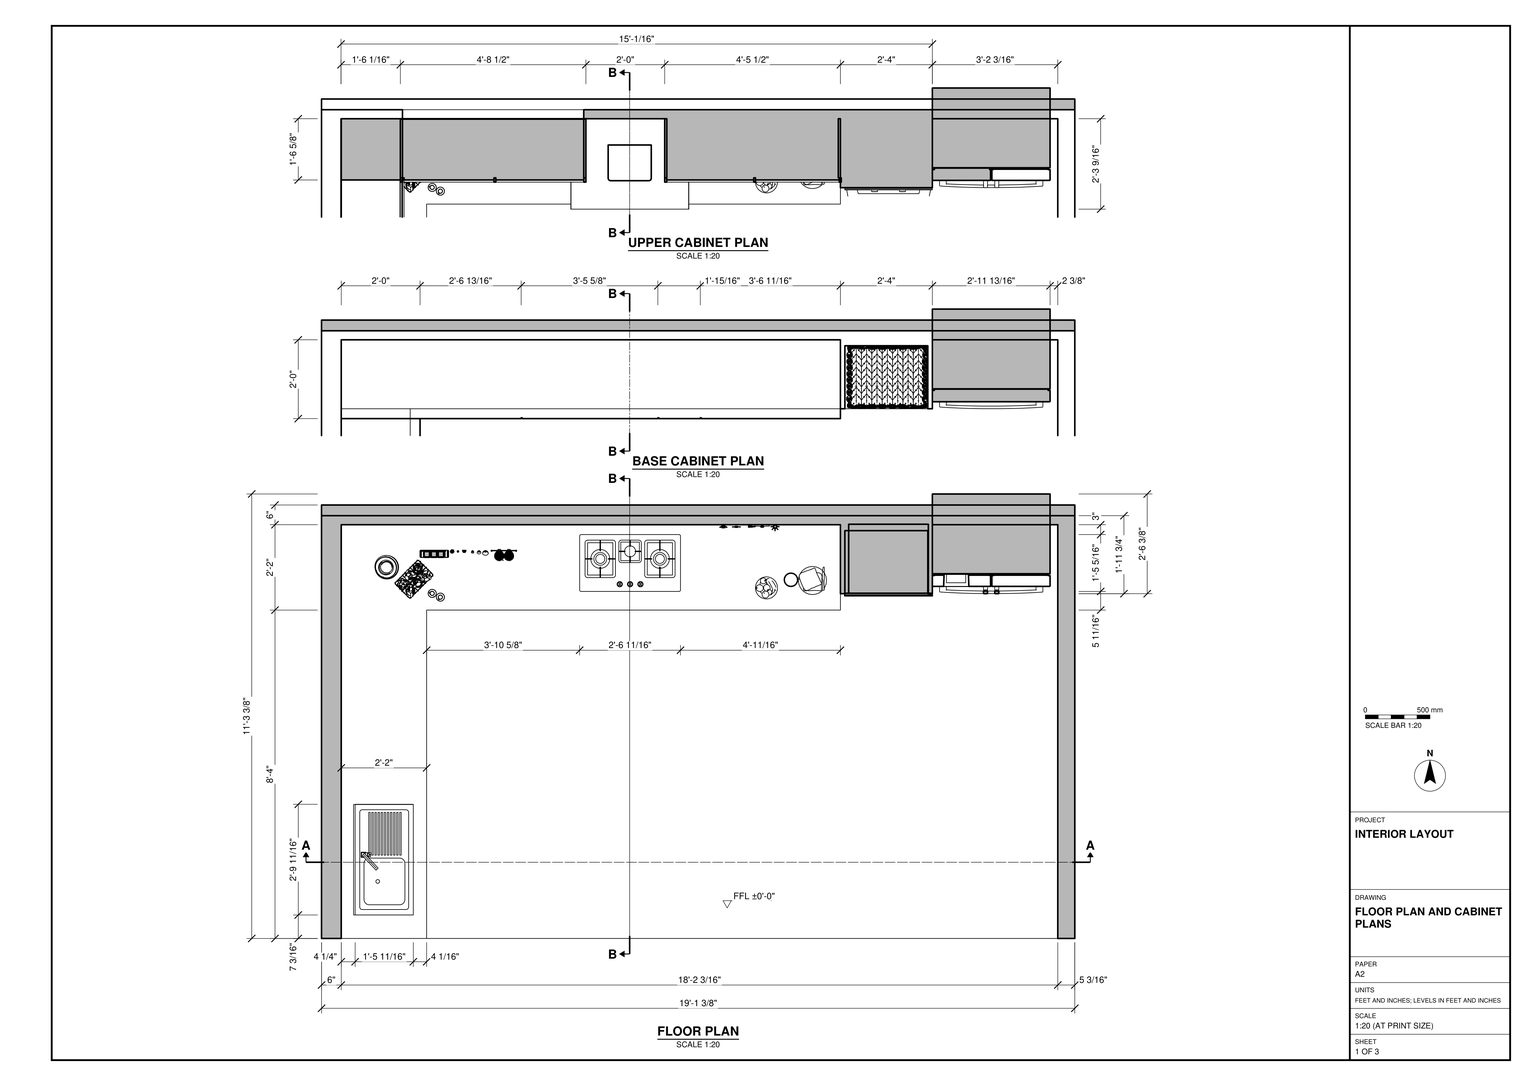
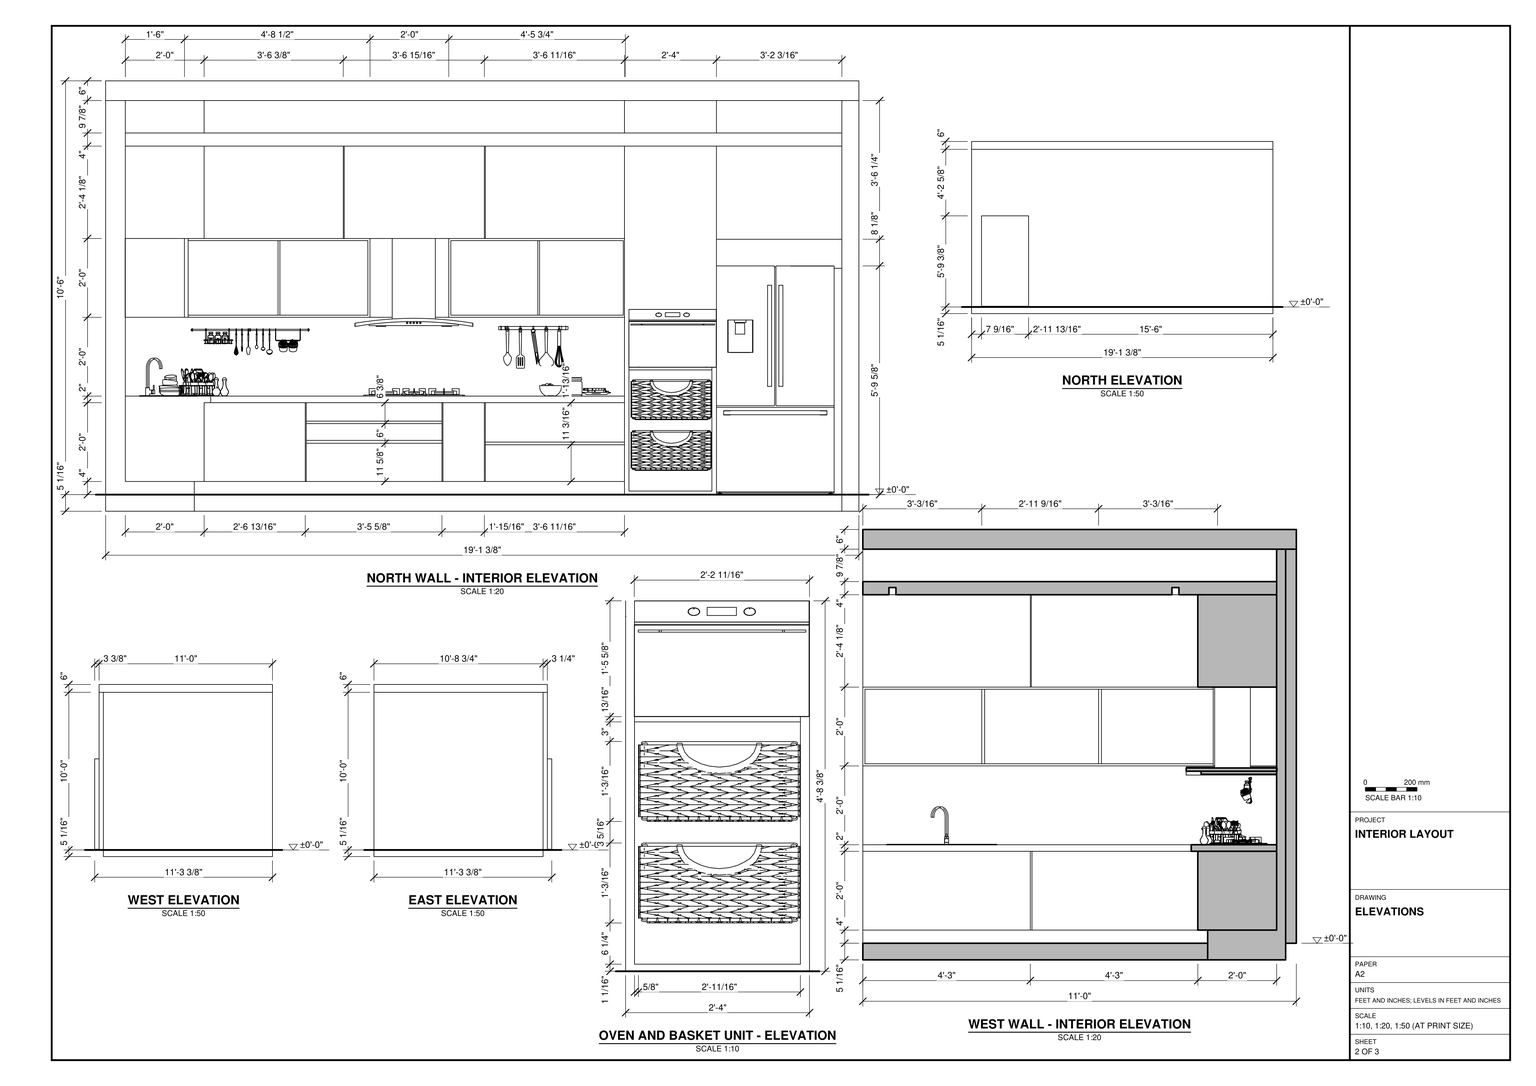
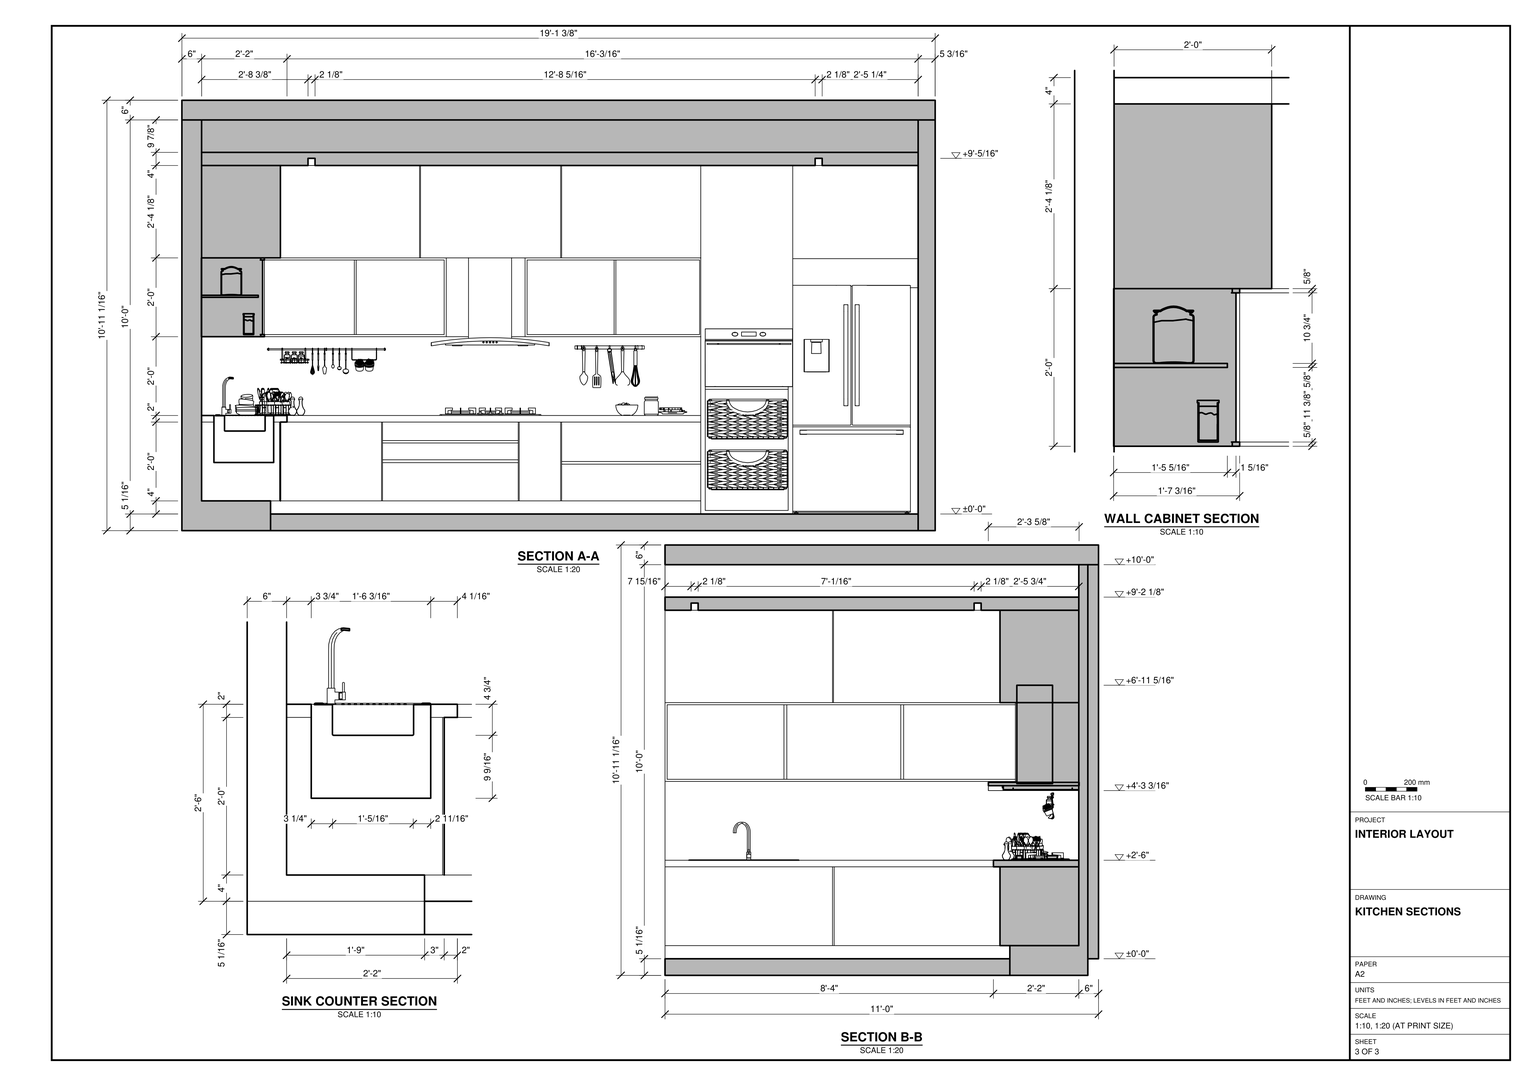
Build the kitchen interior in SketchUp using task_files/diagram_01.pdf. Work in feet and inches. The complete model measures 37'-4 9/16" along X, 24'-8 9/16" along Y and 10'-11 1/16" along Z. Set the finished floor of the single storey at ±0'-0". Use the local plan dimensions for the kitchen itself: the enclosure measures 19'-1 3/8" across the north wall. Model the floor slab, overhead slab, ceiling detail and three enclosing walls at their drawn thicknesses, leaving the south side open as shown.

Fit a continuous L-shaped worktop along the north and west walls. Use the cabinet plans for the depths and the interior elevations for the cupboard fronts, drawer divisions and recessed plinth. Place the sink, draining board and tap near the open end of the west return. Align the cooktop on the north run with the hood in the gap between the wall cabinets. Follow the wall cabinet section for the change in depth between tiers. At the east end of the north run, fit the oven unit with baskets beneath it and place the refrigerator in the adjoining end bay.

Decor and loose items, including appliances, hanging utensils and countertop accessories, may be represented by any suitable library components. Keep shell elements and individual furniture or joinery pieces in separate groups or components, and use components for repeated parts. Save one SketchUp model as output_files/l_shaped_fitted_kitchen_and_its_room_enclosure.skp.

# SketchUp Ruby script. Lengths in inches.
U = 1.inch
M = Sketchup.active_model
def pt(a) = Geom::Point3d.new(a.map { |v| v * U })
def face(e, loops, mat)
  f = e.add_face(loops[0].map { |a| pt(a) })
  loops[1..].each { |l| e.add_face(l.map { |a| pt(a) }).erase! }
  f.material = f.back_material = mat if mat
  f
end
# faces: each face lists its corners as indices into pts; further lists are holes
def faces(e, pts, list, mat = nil) = list.each { |f| face(e, (f[0].is_a?(Array) ? f : [f]).map { |l| l.map { |i| pts[i] } }, mat) }
# xy, xz, yz: faces in a plane at the given z, y or x. An outline is a flat list of corners, or four numbers for a rectangle; further outlines are holes
def ring(l) = l.size == 4 ? [[l[0], l[1]], [l[2], l[1]], [l[2], l[3]], [l[0], l[3]]] : l.each_slice(2).to_a
def flat(e, list, mat, &to3) = list.each { |f| face(e, (f[0].is_a?(Array) ? f : [f]).map { |l| ring(l).map { |u, v| to3.(u, v) } }, mat) }
def xy(e, z, list, mat = nil) = flat(e, list, mat) { |x, y| [x, y, z] }
def xz(e, y, list, mat = nil) = flat(e, list, mat) { |x, z| [x, y, z] }
def yz(e, x, list, mat = nil) = flat(e, list, mat) { |y, z| [x, y, z] }
def lines(e, pts, list) = list.each { |a, b| e.add_line(pt(pts[a]), pt(pts[b])) }
# prism: a flat outline (further loops are holes) pulled along v
def prism(e, loops, v, mat = nil)
  f = face(e, loops, mat); d = Geom::Vector3d.new(v.map { |x| x * U })
  f.pushpull(f.normal.samedirection?(d) ? d.length : -d.length)
end
def box(e, o, s, mat = nil) = prism(e, [[o, [o[0] + s[0], o[1], o[2]], [o[0] + s[0], o[1] + s[1], o[2]], [o[0], o[1] + s[1], o[2]]]], [0, 0, s[2]], mat)
def at(x, y, z, deg = 0) = Geom::Transformation.translation(pt([x, y, z])) * Geom::Transformation.rotation(ORIGIN, Z_AXIS, deg.degrees)
def axes(o, x, y, z) = Geom::Transformation.new([*x, 0, *y, 0, *z, 0, *pt(o).to_a, 1])
def part(name) = M.definitions.add(name)
# library, detail: a bought-in or finely detailed component or shape, given as its bounding box
def library(name, o, s) = part(name).tap { |d| box(d.entities, o, s) }
def detail(e, o, s) = box(e.add_group.entities, o, s)
def put(e, d, t, mat = nil) = e.add_instance(d, t).tap { |i| i.material = mat if mat }
def group(e, t, mat = nil) = e.add_group.tap { |g| g.transformation = t; g.material = mat if mat }.entities
root = M.entities
M.materials.add("[0085_Turquoise]").color = [48, 112, 112]
M.materials.add("[0132_LightGray]").color = [169, 169, 169]
M.materials.add("[0135_DarkGray]").color = [51, 51, 51]
M.materials["[0135_DarkGray]"].alpha = 0.48
M.materials.add("[0136_Charcoal]").color = [33, 33, 33]
M.materials.add("[0136_Charcoal]1").color = [35, 35, 35]
M.materials.add("[0137_Black]").color = [0, 0, 0]
M.materials.add("[Tile Limestone Large]").color = [249, 242, 237]
M.materials.add("[Wax 02]").color = [189, 234, 186]
M.materials.add("cnwhc.com_草图联盟_1kmauOsh").color = [54, 52, 52]
M.materials.add("cnwhc.com_草图联盟_C8Y5Xp2O").color = [156, 156, 156]
M.materials["cnwhc.com_草图联盟_C8Y5Xp2O"].alpha = 0.15
M.materials.add("cnwhc.com_草图联盟_IHFcDxe1").color = [138, 151, 59]
M.materials.add("cnwhc.com_草图联盟_KNEfX85g").color = [162, 126, 87]
M.materials.add("cnwhc.com_草图联盟_QJow1Ky4").color = [144, 133, 65]
M.materials.add("cnwhc.com_草图联盟_z6N5x4Hv").color = [223, 205, 124]
c1 = library("Cup rack\#1",[0,0,0],[12.28,12.62,7.74])
c2 = library("Food+jars (1)",[-3.15,-4.1,0],[15.4,16.05,11.47])
c3 = library("Group\#13",[-397.46,82.38,-0.11],[62.88,62.86,260])
c4 = library("Group\#14",[-282.65,82.375,-0.11],[62.85,62.875,260.02])
c5 = library("Group\#15",[222.96,189.98,-0.44],[259.48,39.25,337.49])
c6 = library("Group\#30",[41.52,-158.49,40.25],[95.93,90.14,172.87])
c7 = library("Group\#21",[-504.125,120.57,-0.1],[108.2,108.21,338.13])
c8 = library("Group\#22",[-376.9,120.94,-0.1],[107.79,107.8,326.37])
c9 = library("Group\#23",[-254.81,120.48,-0.6],[108.21,108.21,334.5])
c10 = library("Group\#24",[-133.01,121.19,-0.1],[106.95,106.95,324.89])
c11 = library("Group\#25",[0.46,121.12,-0.1],[106.94,106.94,338.14])
c12 = library("Group\#26",[151.35,137.54,-0.1],[70.51,70.14,256.45])
c13 = library("Group\#27",[-266.02,-201.27,40.23],[225.02,228.69,89.38])
c14 = library("Group\#28",[-78.56,-74.98,40.25],[131.28,107.59,245.3125])
c15 = library("Group\#31",[-60.55,-181.2,40.41],[105.85,106.35,65.49])
c16 = library("Group\#34",[253.59,42.68,151.97],[53.13,53.13,100.94])
c17 = library("Group\#35",[281.12,-5,151.97],[53.13,53.13,100.92])
c18 = library("Group\#36",[308.75,-52.85,151.97],[53.125,53.13,100.94])
c19 = library("Group\#37",[336.19,-100.38,151.98],[53.13,53.13,100.93])
c20 = library("Group\#38",[363.79,-148.1875,151.98],[53.13,53.13,100.93])
c21 = library("Group\#39",[253.59,42.68,30.7],[53.13,53.13,100.93])
c22 = library("Group\#40",[281.12,-5,30.7],[53.13,53.13,100.91])
c23 = library("Group\#41",[308.75,-52.85,30.7],[53.125,53.13,100.94])
c24 = library("Group\#42",[336.19,-100.38,30.7],[53.13,53.13,100.91])
c25 = library("Group\#43",[363.79,-148.1875,30.7],[53.13,53.13,100.93])
c26 = library("Group\#44",[212.54,-198.04,-0.24],[263.36,352.65,298.47])
c27 = library("Group\#29",[55.69,-19.19,40.37],[80.08,80.05,323.81])
c28 = part("KITCHEN+ITEMS+(1)")
put(c28.entities,c3,at(0,0,0))
put(c28.entities,c4,at(0,0,0))
put(c28.entities,c5,at(0,0,0))
put(c28.entities,c6,at(0,0,-41.3))
put(c28.entities,c7,at(0,0,0))
put(c28.entities,c8,at(0,0,0))
put(c28.entities,c9,at(0,0,0))
put(c28.entities,c10,at(0,0,0))
put(c28.entities,c11,at(0,0,0))
put(c28.entities,c12,at(0,0,0))
put(c28.entities,c13,at(0,0,-41.3))
put(c28.entities,c14,at(0,0,-41.3))
put(c28.entities,c15,at(0,0,-41.3))
put(c28.entities,c16,at(0,0,0))
put(c28.entities,c17,at(0,0,0))
put(c28.entities,c18,at(0,0,0))
put(c28.entities,c19,at(0,0,0))
put(c28.entities,c20,at(0,0,0))
put(c28.entities,c21,at(0,0,0))
put(c28.entities,c22,at(0,0,0))
put(c28.entities,c23,at(0,0,0))
put(c28.entities,c24,at(0,0,0))
put(c28.entities,c25,at(0,0,0))
put(c28.entities,c26,at(0,0,0))
put(c28.entities,c27,at(0,0,-41.3))
c29 = library("Tableware assortment",[-1.93,-1.45,-0.01],[13.28,36.8,12.14])
c30 = library("Food+jars (2)",[-11.5,-3.52,0],[30.82,7.02,10])
c31 = library("Food+jars",[176.18,154.2,55.15],[6.14,23.65,7.76])
c32 = library("Stack of bowls \#1",[0,0,0],[8.98,8.99,10.96])
c33 = library("Oven",[-9.26,-22.59,0.07],[23.42,23.91,23.21])
c34 = library("Library component",[0.34,0,0],[62.86,27.86,1.18])
c35 = library("Woven storage basket",[0,0,0],[10.23,12.78,4.26])
c36 = library("B36CD50SNS_tradeCAD",[0,0,0],[35.84,30.35,69.65])
c37 = library("Bread1",[0,0,0],[12.98,8.57,5.62])
c38 = library("vm_v2_031",[-4.73,-4.73,0],[9.46,9.46,3.85])
c39 = library("Component_12",[0,0,0],[17.72,31.5,20.63])
c40 = library("Kitchen Utensil.",[-24.86,-2.29,-26.5],[81.83,11.85,18.87])
c41 = library("skpC936",[0,-1.9,0],[21.12,3.04,12.85])
c42 = library("PV977NSS_GEProfile",[-17.9375,-27.5625,-0.25],[35.95,27.64,32.08])
c43 = library("Group\#88",[-453.95,-270.9,-0.08],[243.89,243.63,216.82])
c44 = library("Group\#68",[118.34,-437.05,68.8],[33.09,42.97,27.32])
c45 = library("Group\#69",[91.875,-459.8125,1.36],[84.84,84.82,167.94])
c46 = library("Group\#70",[93.63,-458.06,3.28],[81.33,81.31,90.04])
c47 = library("Group\#71",[114.46,-437.1875,150.05],[39.68,39.57,39.67])
c48 = library("Group\#72",[177.52,-496.26,3.28],[81.21,81.23,127.94])
c49 = library("Group\#73",[175.77,-498.01,1.36],[84.71,84.74,167.94])
c50 = library("Group\#74",[198.24,-475.92,149.53],[39.78,40.55,40.71])
c51 = library("Group\#75",[-248.47,-468.28,0.39],[392.05,393.05,278.56])
c52 = library("Group\#76",[-141.57,-278.65,11.2],[96.36,96.33,131.41])
c53 = library("Group\#77",[-62.08,-202.43,11.2],[96.04,96.07,131.41])
c54 = library("Group\#78",[18.13,-280.93,11.2],[96.51,96.54,131.41])
c55 = library("Group\#79",[-213.25,-366.61,11.2],[96.18,96.15,131.41])
c56 = library("Group\#80",[-61.03,-358.93,11.2],[96.54,96.51,131.41])
c57 = library("Group\#81",[8.05,-292.87,22.71],[116.19,111.01,218.49])
c58 = library("Group\#82",[-64.85,-368.89,23],[127.95,108.9,222.0625])
c59 = library("Group\#83",[-143.92,-281.53,22.82],[119.68,105.06,218.38])
c60 = library("Group\#84",[-64.19,-232.55,22.9],[102.65,128.29,224.14])
c61 = library("Group\#85",[-225.25,-376.69,19.19],[116.52,116.69,261.73])
c62 = library("Group\#86",[-138.35,-437.94,11.2],[96.49,96.52,131.41])
c63 = library("Group\#87",[-142.58,-458.38,19.87],[79.66,135.74,256])
c64 = part("KITCHEN+ITEMS+(37)")
put(c64.entities,c43,at(0,0,0))
put(c64.entities,c44,at(0,0,0),"cnwhc.com_草图联盟_IHFcDxe1")
put(c64.entities,c45,at(0,0,0),"cnwhc.com_草图联盟_C8Y5Xp2O")
put(c64.entities,c46,at(0,0,0),"cnwhc.com_草图联盟_QJow1Ky4")
put(c64.entities,c47,at(0,0,0),"cnwhc.com_草图联盟_KNEfX85g")
put(c64.entities,c48,at(0,0,0),"cnwhc.com_草图联盟_z6N5x4Hv")
put(c64.entities,c49,at(0,0,0),"cnwhc.com_草图联盟_C8Y5Xp2O")
put(c64.entities,c50,at(0,0,0),"cnwhc.com_草图联盟_KNEfX85g")
put(c64.entities,c51,at(0,0,0),"cnwhc.com_草图联盟_1kmauOsh")
put(c64.entities,c52,at(0,0,0),"cnwhc.com_草图联盟_C8Y5Xp2O")
put(c64.entities,c53,at(0,0,0),"cnwhc.com_草图联盟_C8Y5Xp2O")
put(c64.entities,c54,at(0,0,0),"cnwhc.com_草图联盟_C8Y5Xp2O")
put(c64.entities,c55,at(0,0,0),"cnwhc.com_草图联盟_C8Y5Xp2O")
put(c64.entities,c56,at(0,0,0),"cnwhc.com_草图联盟_C8Y5Xp2O")
put(c64.entities,c57,at(0,0,0),"cnwhc.com_草图联盟_1kmauOsh")
put(c64.entities,c58,at(0,0,0),"cnwhc.com_草图联盟_1kmauOsh")
put(c64.entities,c59,at(0,0,0),"cnwhc.com_草图联盟_1kmauOsh")
put(c64.entities,c60,at(0,0,0),"cnwhc.com_草图联盟_1kmauOsh")
put(c64.entities,c61,at(0,0,0))
put(c64.entities,c62,at(0,0,0),"cnwhc.com_草图联盟_C8Y5Xp2O")
put(c64.entities,c63,at(0,0,0))
c65 = library("C_HOB (1)",[0,0,0],[30.71,17.32,2.28])
c66 = part("Group\#19")
xy(c66.entities,0,[[0,0,56.49,1.3125]])
xy(c66.entities,0.65,[[0.65,0,28.5,0.66],[28.5,0,29.06,1.3125],[29.06,0,55.85,0.66],[0.65,0.66,28.5,1.3125],[29.06,0.66,55.85,1.3125]])
xy(c66.entities,23.35,[[0.65,0,6,0.66],[6,0,28.5,0.66],[28.5,0,29.06,1.3125],[29.06,0,55.85,0.66],[0.65,0.66,6,1.3125],
  [6,0.66,28.5,1.3125],[29.06,0.66,55.85,1.3125]])
xy(c66.entities,24,[[0,0,6,1.3125],[6,0,56.49,1.3125]])
xz(c66.entities,0,[[[0,0,56.49,24],[0.65,0.65,55.85,23.35]],[28.5,0.65,29.06,23.35]],"[0136_Charcoal]")
xz(c66.entities,0.66,[[0.65,0.65,28.5,23.35],[29.06,0.65,55.85,23.35]],"[0135_DarkGray]")
xz(c66.entities,1.3125,[[[0,0,56.49,24],[0.65,0.65,55.85,23.35]],[28.5,0.65,29.06,23.35]])
yz(c66.entities,0,[[0,0,1.3125,24]])
yz(c66.entities,0.65,[[0.66,0.65,1.3125,11.4],[0.66,11.4,1.3125,12],[0.66,12,1.3125,23.35]])
yz(c66.entities,0.65,[[0,0.65,0.66,11.4],[0,11.4,0.66,12],[0,12,0.66,23.35]],"[0136_Charcoal]")
yz(c66.entities,28.5,[[0.66,0.65,1.3125,23.35]])
yz(c66.entities,28.5,[[0,0.65,0.66,23.35]],"[0136_Charcoal]")
yz(c66.entities,29.06,[[0,0.65,0.66,23.35],[0.66,0.65,1.3125,23.35]])
yz(c66.entities,55.85,[[0.66,0.65,1.3125,11.4],[0.66,11.4,1.3125,12],[0.66,12,1.3125,23.35]])
yz(c66.entities,55.85,[[0,0.65,0.66,11.4],[0,11.4,0.66,12],[0,12,0.66,23.35]],"[0136_Charcoal]")
yz(c66.entities,56.49,[[0,0,1.3125,24]])
xy(root,-5.0625,[[0,0,27,0,27,105,186,105,186,126,224.1875,126,224.1875,0,229.375,0,229.375,128.75,0,128.75]])
xy(root,-5.0625,[[27,0,27,105,186,105,186,126,224.1875,126,224.1875,0]],"[Tile Limestone Large]")
xy(root,0,[[0,128.75,229.375,132]])
xy(root,0,[[27,0,224.1875,0,224.1875,126,186,126,186,105,27,105]],"[Tile Limestone Large]")
xy(root,1.08,[[159.36,105,184.61,124.1875]],"[0136_Charcoal]1")
xy(root,4,[[6,0,27,102],[6,102,27,105],[27,102,27,105,158,105,158,102,115.63,102,115.63,102.25,115.33,102.25,115.33,102,102.72,102,102.72,102.25,102.42,102.25,102.42,102,61.09,102,61.09,102.25,60.79,102.25,60.79,102],[6,105,158,126]])
xy(root,15.6875,[[9.75,7.16,27.94,40.79]])
xy(root,28,[[30,0,30,51,29.75,51,29.75,51.5,30,51.5,30,102,32,102,32,0],[32,100,32,102,60.79,102,60.79,102.25,61.09,102.25,61.09,102,102.42,102,102.42,102.25,102.72,102.25,102.72,102,115.33,102,115.33,102.25,115.63,102.25,115.63,102,158,102,158,100],[6,102,32,126],[32,102,32,126,158,126,158,102,115.63,102,115.63,102.25,115.33,102.25,115.33,102,102.72,102,102.72,102.25,102.42,102.25,102.42,102,61.09,102,61.09,102.25,60.79,102.25,60.79,102]])
xy(root,30,[[[6,0,32,0,32,100,158,100,158,126,6,126],[9.75,7.16,27.94,40.79]]],"[0137_Black]")
xy(root,37.98,[[159.36,105,184.61,124.1875]],"[0136_Charcoal]1")
xy(root,39.33,[[159.36,105,184.61,124.1875]])
xy(root,54,[[5.9375,0,6,126],[6,107.35,24,107.625],[104.49,108,158,126],[24,125.875,80.49,126]])
xy(root,54,[[6,0,24,107.35],[6,107.625,24,126],[24,108,80.49,125.875]],"[0085_Turquoise]")
xy(root,54.65,[[23.875,0.65,24,107.35],[24.65,108,79.85,111.25],[105.14,108,157.35,126],[24.65,111.25,79.85,128.75]])
xy(root,56.07,[[159.36,105,184.61,124.1875]])
xy(root,65.4,[[24.65,108.875,79.85,111.25],[24.65,111.25,79.85,125.875]])
xy(root,66,[[6,0.65,23.25,107.35],[24.65,108.875,79.85,111.25],[105.14,110.3125,157.35,126],[24.65,111.25,79.85,125.875]])
xy(root,66.61,[[6,0.65,23.25,107.35]])
xy(root,66.9,[[105.14,110.3125,157.35,126]])
xy(root,77.35,[[23.875,0.65,24,107.35],[24.65,108,30,111.25],[30,108,79.85,111.25],[105.14,108,157.35,126],[24.65,111.25,30,128.75],
  [30,111.25,79.85,128.75]])
xy(root,77.77,[[186,102,224.1875,126]])
xy(root,78,[[5.9375,0,6,126],[6,0,24,107.35],[6,107.35,24,107.625],[6,107.625,24,126],[24,108,30,125.875],
  [30,108,80.49,125.875],[104.49,108,158,126],[24,125.875,30,126],[30,125.875,80.49,126]])
xy(root,78,[[24,0,24,108,30,108,30,51.3,29.5625,51.3,29.5625,51,30,51,30,0],[30,102,30,108,80.49,108,80.49,126,104.49,126,104.49,108,158,108,158,102,115.63,102,115.63,102.4375,115.33,102.4375,115.33,102,72.67,102,72.67,102.4375,72.37,102.4375,72.37,102]],"[0085_Turquoise]")
xy(root,106.125,[[6,0,6,126,30,126,30,51.3,29.5625,51.3,29.5625,51,30,51,30,0],[30,102,30,126,158,126,158,102,115.63,102,115.63,102.4375,115.33,102.4375,115.33,102,72.67,102,72.67,102.4375,72.37,102.4375,72.37,102],[186,102,224.1875,126],[158,105,186,126]])
xy(root,106.125,[[[30,0,30,51,29.5625,51,29.5625,51.3,30,51.3,30,102,72.37,102,72.37,102.4375,72.67,102.4375,72.67,102,115.33,102,115.33,102.4375,115.63,102.4375,115.63,102,158,102,158,105,186,105,186,102,224.1875,102,224.1875,0],[38.4,7.94,194.96,96.26]],[[40.54,10.08,192.83,94.12],[45.54,85.49,46.48,85.62,47.35,85.98,48.1,86.56,48.68,87.31,49.04,88.18,49.16,89.12,49.04,90.06,48.68,90.93,48.1,91.68,47.35,92.26,46.48,92.62,45.54,92.74,44.6,92.62,43.73,92.26,42.97,91.68,42.4,90.93,42.04,90.06,41.91,89.12,42.04,88.18,42.4,87.31,42.97,86.56,43.73,85.98,44.6,85.62],[45.73,12.08,46.5,12.24,47.2,12.58,47.79,13.1,48.23,13.75,48.48,14.49,48.53,15.27,48.38,16.04,48.04,16.74,47.52,17.33,46.87,17.77,46.13,18.02,45.35,18.07,44.58,17.92,43.875,17.58,43.29,17.0625,42.85,16.41,42.6,15.67,42.54,14.89,42.7,14.12,43.04,13.42,43.56,12.83,44.21,12.39,44.95,12.14],[187.83,86.2,188.58,86.3,189.29,86.59,189.89,87.05,190.36,87.66,190.65,88.36,190.75,89.12,190.65,89.875,190.36,90.58,189.89,91.18,189.29,91.65,188.58,91.94,187.83,92.04,187.07,91.94,186.37,91.65,185.76,91.18,185.3,90.58,185.01,89.875,184.91,89.12,185.01,88.36,185.3,87.66,185.76,87.05,186.37,86.59,187.07,86.3],[187.83,12.64,188.46,12.72,189.05,12.97,189.55,13.36,189.94,13.86,190.18,14.45,190.27,15.08,190.18,15.71,189.94,16.3,189.55,16.8,189.05,17.19,188.46,17.43,187.83,17.52,187.2,17.43,186.61,17.19,186.11,16.8,185.72,16.3,185.47,15.71,185.39,15.08,185.47,14.45,185.72,13.86,186.11,13.36,186.61,12.97,187.2,12.72]]],"[0132_LightGray]")
xy(root,107.375,[[45.73,12.08,44.95,12.14,44.21,12.39,43.56,12.83,43.04,13.42,42.7,14.12,42.54,14.89,42.6,15.67,42.85,16.41,43.29,17.0625,43.875,17.58,44.58,17.92,45.35,18.07,46.13,18.02,46.87,17.77,47.52,17.33,48.04,16.74,48.38,16.04,48.53,15.27,48.48,14.49,48.23,13.75,47.79,13.1,47.2,12.58,46.5,12.24],[187.83,12.64,187.2,12.72,186.61,12.97,186.11,13.36,185.72,13.86,185.47,14.45,185.39,15.08,185.47,15.71,185.72,16.3,186.11,16.8,186.61,17.19,187.2,17.43,187.83,17.52,188.46,17.43,189.05,17.19,189.55,16.8,189.94,16.3,190.18,15.71,190.27,15.08,190.18,14.45,189.94,13.86,189.55,13.36,189.05,12.97,188.46,12.72],[45.54,85.49,44.6,85.62,43.73,85.98,42.97,86.56,42.4,87.31,42.04,88.18,41.91,89.12,42.04,90.06,42.4,90.93,42.97,91.68,43.73,92.26,44.6,92.62,45.54,92.74,46.48,92.62,47.35,92.26,48.1,91.68,48.68,90.93,49.04,90.06,49.16,89.12,49.04,88.18,48.68,87.31,48.1,86.56,47.35,85.98,46.48,85.62],[187.83,86.2,187.07,86.3,186.37,86.59,185.76,87.05,185.3,87.66,185.01,88.36,184.91,89.12,185.01,89.875,185.3,90.58,185.76,91.18,186.37,91.65,187.07,91.94,187.83,92.04,188.58,91.94,189.29,91.65,189.89,91.18,190.36,90.58,190.65,89.875,190.75,89.12,190.65,88.36,190.36,87.66,189.89,87.05,189.29,86.59,188.58,86.3]])
xy(root,108.3125,[[[38.4,7.94,194.96,96.26],[40.54,10.08,192.83,94.12]]])
xy(root,110.125,[[6,0,224.1875,126]])
xy(root,120,[[0,0,0,128.75,229.375,128.75,229.375,0,224.1875,0,224.1875,126,6,126,6,0],[6,0,224.1875,126],[0,128.75,229.375,132]])
xy(root,126,[[0,0,229.375,132]])
xz(root,0,[[0,-5.0625,27,-5.0625,27,4,6,4,6,54,5.9375,54,5.9375,78,6,78,6,120,0,120],[224.1875,-5.0625,229.375,120],[5.9375,54,6,78],[6,106.125,224.1875,110.125],[0,120,229.375,126]])
xz(root,0,[[6,54,24,78],[6,78,30,106.125]],"[0085_Turquoise]")
xz(root,0,[[6,4,30,4,30,28,32,28,32,30,6,30]],"[0137_Black]")
xz(root,0,[[27,-5.0625,224.1875,0]],"[Tile Limestone Large]")
xz(root,0.65,[[23.875,54.65,24,54.65,24,77.35,23.875,77.35,23.875,66.61,23.25,66.61,23.25,66,23.875,66],[6,66,23.25,66.61]])
xz(root,7.16,[[9.75,15.6875,27.94,30]])
xz(root,7.94,[[38.4,106.125,194.96,108.3125]])
xz(root,10.08,[[40.54,106.125,192.83,108.3125]])
xz(root,40.79,[[9.75,15.6875,27.94,30]])
xz(root,51,[[29.75,4,30,28],[29.5625,78,30,106.125]])
xz(root,51.3,[[29.5625,78,30,106.125]])
xz(root,51.5,[[29.75,4,30,28]])
xz(root,94.12,[[40.54,106.125,192.83,108.3125]])
xz(root,96.26,[[38.4,106.125,194.96,108.3125]])
xz(root,100,[[32,28,158,30]],"[0137_Black]")
xz(root,102,[[6,4,30,28]])
xz(root,102,[[30,4,60.79,28],[61.09,4,102.42,15.65],[102.72,4,115.33,28],[115.63,4,158,15.18],[115.63,16,158,28],
  [61.09,16.52,102.42,21.63],[61.09,22.375,102.42,28],[186,77.77,224.1875,106.125],[30,78,72.37,106.125],[72.67,78,115.33,106.125],
  [115.63,78,158,106.125]],"[0085_Turquoise]")
xz(root,102,[[115.63,15.18,158,16],[61.09,15.65,102.42,16.52],[61.09,21.63,102.42,22.375]],"[0136_Charcoal]1")
xz(root,102.25,[[60.79,4,61.09,28],[102.42,4,102.72,28],[115.33,4,115.63,28]])
xz(root,102.4375,[[72.37,78,72.67,106.125],[115.33,78,115.63,106.125]])
xz(root,105,[[158,-5.0625,186,0],[[158,0,186,106.125],[159.36,1.08,184.61,56.07]],[159.36,37.98,184.61,39.33]],"[0085_Turquoise]")
xz(root,105,[[27,-5.0625,158,0],[27,0,158,4]],"[0136_Charcoal]1")
xz(root,107.35,[[6,54,24,54,24,54.65,23.875,54.65,23.875,66,6,66],[23.875,54.65,24,54.65,24,77.35,23.875,77.35,23.875,66.61,23.25,66.61,23.25,66,23.875,66],[6,66,23.25,66.61],[6,66.61,23.875,66.61,23.875,77.35,24,77.35,24,78,6,78]])
xz(root,108,[[[24,54,80.49,78],[24.65,54.65,79.85,77.35]],[[104.49,54,158,78],[105.14,54.65,157.35,77.35]]])
xz(root,108.875,[[24.65,65.4,79.85,66]])
xz(root,110.3125,[[105.14,66,157.35,66.9]])
xz(root,111.25,[[24.65,65.4,79.85,66]])
xz(root,124.1875,[[159.36,39.33,184.61,56.07]])
xz(root,124.1875,[[159.36,1.08,184.61,37.98]],"[0136_Charcoal]1")
xz(root,125.875,[[24,54,80.49,78],[24.65,65.4,79.85,66]])
xz(root,126,[[186,-5.0625,224.1875,0],[186,0,224.1875,68.91],[6,4,158,28],[6,28,32,30],[32,28,160,30],
  [5.9375,54,6,78],[6,54,24,78],[24,54,80.49,78],[80.49,54,104.49,78],[[104.49,54,158,78],[105.14,54.65,157.35,77.35]],
  [105.14,66,157.35,66.9],[186,68.91,224.1875,77.77],[6,78,30,106.125],[30,78,158,106.125],[6,106.125,30,110.125],
  [30,106.125,158,110.125],[158,106.125,186,110.125],[186,106.125,224.1875,110.125],[6,110.125,30,120],[30,110.125,158,120],
  [158,110.125,186,120],[186,110.125,224.1875,120]])
xz(root,126,[[6,30,158,54]],"[Wax 02]")
xz(root,128.75,[[0,-5.0625,229.375,0],[[0,0,229.375,120],[24.65,54.65,79.85,77.35]]])
xz(root,132,[[0,0,229.375,120],[0,120,229.375,126]])
yz(root,0,[[0,-5.0625,128.75,120],[128.75,0,132,120],[0,120,132,126]])
yz(root,5.9375,[[0,54,126,78]])
yz(root,6,[[0,4,0,30,126,30,126,28,102,28,102,4],[102,4,126,28],[0,54,107.35,54,107.35,66,0.65,66,0.65,66.61,107.35,66.61,107.35,78,0,78],[107.35,54,107.625,78],[107.625,54,126,78],
  [0.65,66,107.35,66.61],[0,78,126,106.125],[0,106.125,126,110.125],[0,110.125,126,120]])
yz(root,6,[[0,30,126,54]],"[Wax 02]")
yz(root,9.75,[[7.16,15.6875,40.79,30]])
yz(root,23.25,[[0.65,66,107.35,66.61]])
yz(root,24,[[0,54,107.35,54,107.35,54.65,0.65,54.65,0.65,77.35,107.35,77.35,107.35,78,0,78],[107.35,54,108,78],[108,54,125.875,78],[125.875,54,126,78]])
yz(root,24.65,[[108,54.65,111.25,65.4],[111.25,54.65,128.75,54.65,128.75,77.35,111.25,77.35,111.25,66,125.875,66,125.875,65.4,111.25,65.4],[108,65.4,108.875,66],[108.875,65.4,111.25,66],[108,66,111.25,77.35]])
yz(root,27,[[0,-5.0625,105,0],[0,0,105,4]],"[0136_Charcoal]1")
yz(root,27.94,[[7.16,15.6875,40.79,30]])
yz(root,29.5625,[[51,78,51.3,106.125]])
yz(root,29.75,[[51,4,51.5,28]])
yz(root,30,[[102,78,126,106.125]])
yz(root,30,[[0,4,51,28],[51.5,4,102,28],[0,78,51,106.125],[51.3,78,102,106.125]],"[0085_Turquoise]")
yz(root,32,[[0,28,100,30]],"[0137_Black]")
yz(root,38.4,[[7.94,106.125,96.26,108.3125]])
yz(root,40.54,[[10.08,106.125,94.12,108.3125]])
yz(root,60.79,[[102,4,102.25,28]])
yz(root,61.09,[[102,4,102.25,28]])
yz(root,72.37,[[102,78,102.4375,106.125]])
yz(root,72.67,[[102,78,102.4375,106.125]])
yz(root,79.85,[[108,54.65,111.25,65.4],[111.25,54.65,111.25,65.4,125.875,65.4,125.875,66,111.25,66,111.25,77.35,128.75,77.35,128.75,54.65],[108,65.4,108.875,66],[108.875,65.4,111.25,66],[108,66,111.25,77.35]])
yz(root,80.49,[[108,54,125.875,78],[125.875,54,126,78]])
yz(root,102.42,[[102,4,102.25,28]])
yz(root,102.72,[[102,4,102.25,28]])
yz(root,104.49,[[108,54,126,78]])
yz(root,105.14,[[108,54.65,126,66],[108,66,110.3125,66.9],[110.3125,66,126,66.9],[108,66.9,126,77.35]])
yz(root,115.33,[[102,4,102.25,28],[102,78,102.4375,106.125]])
yz(root,115.63,[[102,4,102.25,28],[102,78,102.4375,106.125]])
yz(root,157.35,[[108,54.65,126,66],[108,66,110.3125,66.9],[110.3125,66,126,66.9],[108,66.9,126,77.35]])
yz(root,158,[[102,4,105,28],[105,4,126,28],[100,28,105,30],[105,30,126,54],[105,54,108,78],
  [108,54,126,78],[102,78,105,106.125],[105,78,126,106.125]])
yz(root,159.36,[[105,39.33,124.1875,56.07]])
yz(root,159.36,[[105,1.08,124.1875,37.98]],"[0136_Charcoal]1")
yz(root,184.61,[[105,39.33,124.1875,56.07]])
yz(root,184.61,[[105,1.08,124.1875,37.98]],"[0136_Charcoal]1")
yz(root,186,[[105,-5.0625,126,0],[105,0,126,68.91],[105,68.91,126,77.77],[102,77.77,105,106.125]])
yz(root,192.83,[[10.08,106.125,94.12,108.3125]])
yz(root,194.96,[[7.94,106.125,96.26,108.3125]])
yz(root,224.1875,[[0,106.125,126,110.125],[0,110.125,126,120]])
yz(root,224.1875,[[0,-5.0625,126,0],[0,0,126,0,126,77.77,102,77.77,102,106.125,0,106.125]],"[0132_LightGray]")
yz(root,229.375,[[0,-5.0625,128.75,120],[128.75,0,132,120],[0,120,132,126]])
p = [[44.95,12.14,106.125],[44.21,12.39,106.125],[44.21,12.39,107.375],[44.95,12.14,107.375],[45.73,12.08,106.125],[45.73,12.08,107.375],
  [46.5,12.24,106.125],[46.5,12.24,107.375],[47.2,12.58,106.125],[47.2,12.58,107.375],[43.56,12.83,106.125],[43.56,12.83,107.375],
  [47.79,13.1,106.125],[47.79,13.1,107.375],[187.83,12.64,106.125],[187.2,12.72,106.125],[187.2,12.72,107.375],[187.83,12.64,107.375],
  [188.46,12.72,106.125],[188.46,12.72,107.375],[186.61,12.97,106.125],[186.61,12.97,107.375],[189.05,12.97,106.125],[189.05,12.97,107.375],
  [43.04,13.42,106.125],[43.04,13.42,107.375],[186.11,13.36,106.125],[186.11,13.36,107.375],[189.55,13.36,106.125],[189.55,13.36,107.375],
  [48.23,13.75,106.125],[48.23,13.75,107.375],[42.7,14.12,106.125],[42.7,14.12,107.375],[185.72,13.86,106.125],[185.72,13.86,107.375],
  [189.94,13.86,106.125],[189.94,13.86,107.375],[48.48,14.49,106.125],[48.48,14.49,107.375],[185.47,14.45,106.125],[185.47,14.45,107.375],
  [190.18,14.45,106.125],[190.18,14.45,107.375],[42.54,14.89,106.125],[42.54,14.89,107.375],[185.39,15.08,106.125],[185.39,15.08,107.375],
  [190.27,15.08,106.125],[190.27,15.08,107.375],[48.53,15.27,106.125],[48.53,15.27,107.375],[42.6,15.67,106.125],[42.6,15.67,107.375],
  [185.47,15.71,106.125],[185.47,15.71,107.375],[190.18,15.71,106.125],[190.18,15.71,107.375],[48.38,16.04,106.125],[48.38,16.04,107.375],
  [42.85,16.41,106.125],[42.85,16.41,107.375],[185.72,16.3,106.125],[185.72,16.3,107.375],[189.94,16.3,106.125],[189.94,16.3,107.375],
  [48.04,16.74,106.125],[48.04,16.74,107.375],[186.11,16.8,106.125],[186.11,16.8,107.375],[189.55,16.8,106.125],[189.55,16.8,107.375],
  [43.29,17.0625,106.125],[43.29,17.0625,107.375],[47.52,17.33,106.125],[47.52,17.33,107.375],[186.61,17.19,106.125],[186.61,17.19,107.375],
  [189.05,17.19,106.125],[189.05,17.19,107.375],[43.875,17.58,106.125],[43.875,17.58,107.375],[187.2,17.43,106.125],[187.2,17.43,107.375],
  [188.46,17.43,106.125],[188.46,17.43,107.375],[46.87,17.77,106.125],[46.87,17.77,107.375],[187.83,17.52,106.125],[187.83,17.52,107.375],
  [44.58,17.92,106.125],[44.58,17.92,107.375],[46.13,18.02,106.125],[46.13,18.02,107.375],[45.35,18.07,106.125],[45.35,18.07,107.375],
  [45.54,85.49,106.125],[44.6,85.62,106.125],[44.6,85.62,107.375],[45.54,85.49,107.375],[46.48,85.62,106.125],[46.48,85.62,107.375],
  [43.73,85.98,106.125],[43.73,85.98,107.375],[47.35,85.98,106.125],[47.35,85.98,107.375],[42.97,86.56,106.125],[42.97,86.56,107.375],
  [48.1,86.56,106.125],[48.1,86.56,107.375],[187.83,86.2,106.125],[187.07,86.3,106.125],[187.07,86.3,107.375],[187.83,86.2,107.375],
  [188.58,86.3,106.125],[188.58,86.3,107.375],[186.37,86.59,106.125],[186.37,86.59,107.375],[189.29,86.59,106.125],[189.29,86.59,107.375],
  [42.4,87.31,106.125],[42.4,87.31,107.375],[48.68,87.31,106.125],[48.68,87.31,107.375],[185.76,87.05,106.125],[185.76,87.05,107.375],
  [189.89,87.05,106.125],[189.89,87.05,107.375],[185.3,87.66,106.125],[185.3,87.66,107.375],[190.36,87.66,106.125],[190.36,87.66,107.375],
  [42.04,88.18,106.125],[42.04,88.18,107.375],[49.04,88.18,106.125],[49.04,88.18,107.375],[185.01,88.36,106.125],[185.01,88.36,107.375],
  [190.65,88.36,106.125],[190.65,88.36,107.375],[41.91,89.12,106.125],[41.91,89.12,107.375],[49.16,89.12,106.125],[49.16,89.12,107.375],
  [184.91,89.12,106.125],[184.91,89.12,107.375],[190.75,89.12,106.125],[190.75,89.12,107.375],[42.04,90.06,106.125],[42.04,90.06,107.375],
  [49.04,90.06,106.125],[49.04,90.06,107.375],[185.01,89.875,106.125],[185.01,89.875,107.375],[190.65,89.875,106.125],[190.65,89.875,107.375],
  [185.3,90.58,106.125],[185.3,90.58,107.375],[190.36,90.58,106.125],[190.36,90.58,107.375],[42.4,90.93,106.125],[42.4,90.93,107.375],
  [48.68,90.93,106.125],[48.68,90.93,107.375],[185.76,91.18,106.125],[185.76,91.18,107.375],[189.89,91.18,106.125],[189.89,91.18,107.375],
  [42.97,91.68,106.125],[42.97,91.68,107.375],[48.1,91.68,106.125],[48.1,91.68,107.375],[186.37,91.65,106.125],[186.37,91.65,107.375],
  [189.29,91.65,106.125],[189.29,91.65,107.375],[187.07,91.94,106.125],[187.07,91.94,107.375],[188.58,91.94,106.125],[188.58,91.94,107.375],
  [43.73,92.26,106.125],[43.73,92.26,107.375],[47.35,92.26,106.125],[47.35,92.26,107.375],[187.83,92.04,106.125],[187.83,92.04,107.375],
  [44.6,92.62,106.125],[44.6,92.62,107.375],[46.48,92.62,106.125],[46.48,92.62,107.375],[45.54,92.74,106.125],[45.54,92.74,107.375],
  [160,126,28],[160,105,28],[384.625,-201.2,83.74],[385.625,-201.2,83.74],[385.625,-200.2,83.74]]
faces(root,p,[[0,1,2,3],[4,0,3,5],[6,4,5,7],[8,6,7,9],[1,10,11,2],[12,8,9,13],[14,15,16,17],[18,14,17,19],
  [15,20,21,16],[22,18,19,23],[10,24,25,11],[20,26,27,21],[28,22,23,29],[30,12,13,31],[24,32,33,25],[26,34,35,27],
  [36,28,29,37],[38,30,31,39],[34,40,41,35],[42,36,37,43],[32,44,45,33],[40,46,47,41],[48,42,43,49],[50,38,39,51],
  [44,52,53,45],[46,54,55,47],[56,48,49,57],[58,50,51,59],[52,60,61,53],[54,62,63,55],[64,56,57,65],[66,58,59,67],
  [62,68,69,63],[70,64,65,71],[60,72,73,61],[74,66,67,75],[68,76,77,69],[78,70,71,79],[72,80,81,73],[76,82,83,77],
  [84,78,79,85],[86,74,75,87],[82,88,89,83],[88,84,85,89],[80,90,91,81],[92,86,87,93],[90,94,95,91],[94,92,93,95],
  [96,97,98,99],[100,96,99,101],[97,102,103,98],[104,100,101,105],[102,106,107,103],[108,104,105,109],[110,111,112,113],[114,110,113,115],
  [111,116,117,112],[118,114,115,119],[106,120,121,107],[122,108,109,123],[116,124,125,117],[126,118,119,127],[124,128,129,125],[130,126,127,131],
  [120,132,133,121],[134,122,123,135],[128,136,137,129],[138,130,131,139],[132,140,141,133],[142,134,135,143],[136,144,145,137],[146,138,139,147],
  [140,148,149,141],[150,142,143,151],[144,152,153,145],[154,146,147,155],[152,156,157,153],[158,154,155,159],[148,160,161,149],[162,150,151,163],
  [156,164,165,157],[166,158,159,167],[160,168,169,161],[170,162,163,171],[164,172,173,165],[174,166,167,175],[172,176,177,173],[178,174,175,179],
  [168,180,181,169],[182,170,171,183],[176,184,185,177],[184,178,179,185],[180,186,187,181],[188,182,183,189],[186,190,191,187],[190,188,189,191]])
lines(root,p,[[192,193],[194,195],[195,196],[196,194]])
put(root,c1,at(123.74,110.125,54.65))
put(root,c2,axes([143.08,113,54.65],[0.67,0,0],[0,0.67,0],[0,0,0.67]))
put(root,c28,axes([129.25,117.85,66.93],[0.03637,0,0],[0,0.0166,0],[0,0,0.02636]))
put(root,c29,axes([69.62,112.68,54.65],[0,0.74,0],[-0.851,0,0],[0,0,0.74]))
put(root,c30,at(47.72,116.42,66))
put(root,c31,at(200.18,250.125,-0.5,-180))
put(root,c31,at(200.18,222.9375,-0.5,-180))
put(root,c31,at(200.18,191.5,-0.5,-180))
put(root,c32,axes([12.5,5.68,66.61],[0.8288,0,0],[0,0.8288,0],[0,0,0.8288]))
put(root,c30,at(15.05,29.62,66.61,90))
put(root,c30,at(15.05,68.05,66.61,90))
put(root,c33,axes([169.87,124.82,38.71],[1.13886,0,0],[0,1,0],[0,0,0.76]))
put(root,c34,at(385.375,-161.24,83.23))
put(root,c35,axes([159.96,105.14,22.8125],[2.41,0,0],[0,1.49,0],[0,0,2.8574]))
put(root,c35,axes([159.96,105,7.36],[2.41,0,0],[0,1.49,0],[0,0,2.8574]))
put(root,c36,at(186,105,0))
put(root,c37,at(140.8,104.72,30))
put(root,c38,at(135.48,106.77,30))
put(root,c39,axes([10.23,7.16,20.96],[1,0,0],[0,1.07,0],[0,0,1]))
put(root,c40,axes([51.08,118.35,53.99],[-0.44,0,0],[0,-0.44,0],[0,0,0.44]))
put(root,c41,at(119.68,126,38.48))
put(root,c42,at(93.84,126,51.46))
put(root,c64,axes([29.71,117.48,30],[0.0297,0,0],[0,0.0297,0],[0,0,0.0297]))
put(root,c65,at(78.6,105.68,30))
g1 = group(root,at(24,0,54))
xy(g1,0,[[0,0,1.125,107.35],[0,107.35,1.125,107.625],[0,107.625,1.125,108]])
xy(g1,0.65,[[0,0.65,0.5625,36.22],[0,36.22,1.125,37.09],[0,37.09,0.5625,71.78],[0,71.78,1.125,72.66],[0,72.66,0.5625,107.35]])
xy(g1,0.65,[[0.5625,0.65,1.125,36.22],[0.5625,37.09,1.125,71.78],[0.5625,72.66,1.125,107.35]],"[0136_Charcoal]")
xy(g1,23.35,[[0,0.65,0.5625,36.22],[0.5625,0.65,1.125,36.22],[0,36.22,1.125,37.09],[0,37.09,0.5625,71.78],[0.5625,37.09,1.125,71.78],
  [0,71.78,1.125,72.66],[0,72.66,0.5625,107.35],[0.5625,72.66,1.125,107.35]])
xy(g1,24,[[0,107.35,1.125,107.625],[0,107.625,1.125,108]])
xy(g1,24,[[0,0,1.125,107.35]],"[0136_Charcoal]")
xz(g1,0,[[0,0,1.125,24]],"[0136_Charcoal]")
xz(g1,0.65,[[0,0.65,0.5625,23.35],[0.5625,0.65,1.125,23.35]])
xz(g1,36.22,[[0,0.65,0.5625,23.35]])
xz(g1,36.22,[[0.5625,0.65,1.125,23.35]],"[0136_Charcoal]")
xz(g1,37.09,[[0,0.65,0.5625,23.35],[0.5625,0.65,1.125,23.35]])
xz(g1,71.78,[[0,0.65,0.5625,23.35]])
xz(g1,71.78,[[0.5625,0.65,1.125,23.35]],"[0136_Charcoal]")
xz(g1,72.66,[[0,0.65,0.5625,23.35],[0.5625,0.65,1.125,23.35]])
xz(g1,107.35,[[0,0.65,0.5625,23.35]])
xz(g1,107.35,[[0.5625,0.65,1.125,23.35]],"[0136_Charcoal]")
xz(g1,108,[[0,0,1.125,24]])
yz(g1,0,[[107.35,0,108,24],[36.22,0.65,37.09,23.35],[71.78,0.65,72.66,23.35]])
yz(g1,0.5625,[[0.65,0.65,36.22,23.35],[37.09,0.65,71.78,23.35],[72.66,0.65,107.35,23.35]],"[0135_DarkGray]")
yz(g1,1.125,[[0,0,107.35,0,107.35,0.65,0.65,0.65,0.65,23.35,107.35,23.35,107.35,24,0,24],[107.35,0,108,24],[36.22,0.65,37.09,23.35],[71.78,0.65,72.66,23.35]],"[0136_Charcoal]")
put(root,c66,at(24.01,106.6875,54))
put(root,c66,axes([104.49,106.6875,54],[0.95165,0,0],[0,1,0],[0,0,1]))
